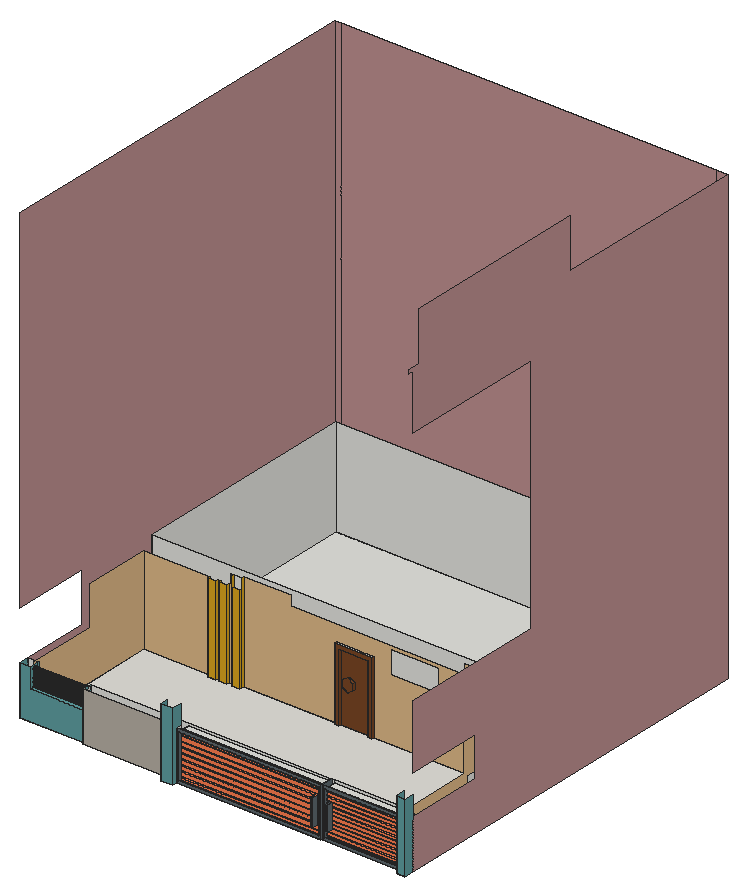
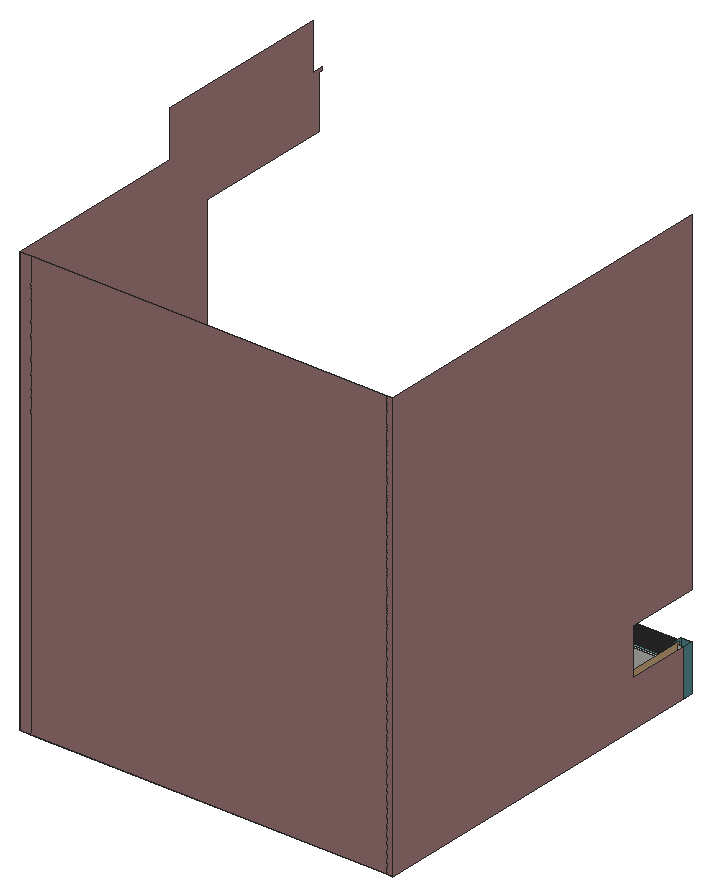
# SketchUp Ruby script. Lengths in inches.
U = 1.inch
M = Sketchup.active_model
def pt(a) = Geom::Point3d.new(a.map { |v| v * U })
def face(e, loops, mat)
  f = e.add_face(loops[0].map { |a| pt(a) })
  loops[1..].each { |l| e.add_face(l.map { |a| pt(a) }).erase! }
  f.material = f.back_material = mat if mat
  f
end
# faces: each face lists its corners as indices into pts; further lists are holes
def faces(e, pts, list, mat = nil) = list.each { |f| face(e, (f[0].is_a?(Array) ? f : [f]).map { |l| l.map { |i| pts[i] } }, mat) }
# xy, xz, yz: faces in a plane at the given z, y or x. An outline is a flat list of corners, or four numbers for a rectangle; further outlines are holes
def ring(l) = l.size == 4 ? [[l[0], l[1]], [l[2], l[1]], [l[2], l[3]], [l[0], l[3]]] : l.each_slice(2).to_a
def flat(e, list, mat, &to3) = list.each { |f| face(e, (f[0].is_a?(Array) ? f : [f]).map { |l| ring(l).map { |u, v| to3.(u, v) } }, mat) }
def xy(e, z, list, mat = nil) = flat(e, list, mat) { |x, y| [x, y, z] }
def xz(e, y, list, mat = nil) = flat(e, list, mat) { |x, z| [x, y, z] }
def yz(e, x, list, mat = nil) = flat(e, list, mat) { |y, z| [x, y, z] }
def lines(e, pts, list) = list.each { |a, b| e.add_line(pt(pts[a]), pt(pts[b])) }
# prism: a flat outline (further loops are holes) pulled along v
def prism(e, loops, v, mat = nil)
  f = face(e, loops, mat); d = Geom::Vector3d.new(v.map { |x| x * U })
  f.pushpull(f.normal.samedirection?(d) ? d.length : -d.length)
end
def box(e, o, s, mat = nil) = prism(e, [[o, [o[0] + s[0], o[1], o[2]], [o[0] + s[0], o[1] + s[1], o[2]], [o[0], o[1] + s[1], o[2]]]], [0, 0, s[2]], mat)
def at(x, y, z, deg = 0) = Geom::Transformation.translation(pt([x, y, z])) * Geom::Transformation.rotation(ORIGIN, Z_AXIS, deg.degrees)
def axes(o, x, y, z) = Geom::Transformation.new([*x, 0, *y, 0, *z, 0, *pt(o).to_a, 1])
def part(name) = M.definitions.add(name)
# library, detail: a bought-in or finely detailed component or shape, given as its bounding box
def library(name, o, s) = part(name).tap { |d| box(d.entities, o, s) }
def detail(e, o, s) = box(e.add_group.entities, o, s)
def put(e, d, t, mat = nil) = e.add_instance(d, t).tap { |i| i.material = mat if mat }
def group(e, t, mat = nil) = e.add_group.tap { |g| g.transformation = t; g.material = mat if mat }.entities
root = M.entities
M.materials.add("[0025_Coral]").color = [255, 127, 80]
M.materials.add("[0036_BurlyWood]").color = [222, 184, 135]
M.materials.add("[0045_Goldenrod]").color = [218, 165, 32]
M.materials.add("[0081_CadetBlue]").color = [95, 158, 160]
M.materials.add("[0119_RosyBrown]").color = [188, 143, 143]
M.materials.add("[Color M07]").color = [58, 58, 58]
M.materials.add("[Formica Speckled Grey]").color = [94, 105, 111]
M.materials.add("[Marble Carrara Gold Floor Tile]").color = [225, 223, 217]
M.materials.add("[Stone Masonry Multi]").color = [182, 175, 164]
M.materials.add("[Translucent Glass Blue]").color = [100, 149, 237]
M.materials["[Translucent Glass Blue]"].alpha = 0.5
M.materials.add("[Wood Floor Parquet]").color = [145, 89, 39]
M.materials.add("[Wood Veneer 01]").color = [120, 70, 37]
xy(root,0,[[181.875,0,195.69,12],[469.21,0,471,12],[471,0,480,12],[373.99,6,374.05,12],[79.49,9,181.875,11.375],
  [79.49,11.375,181.875,12],[0,12,79.49,24.5],[372.4375,12,373.99,21],[373.99,12,376.99,21],[466.21,12,466.21,21,471,21,471,18.5625,469.21,18.5625,469.21,12],
  [469.21,12,471,18.5625],[471,12,480,18.5625],[471,18.5625,480,106.65],[0,24.5,9,106.65],[0,106.65,7.75,492],
  [7.75,106.65,7.75,492,466.21,492,466.21,483,9,483,9,201.23,466.21,201.23,466.21,192.3,129,192.3,129,189.3,113.21,189.3,113.21,186.3,103.48,186.3,103.48,189.3,99.83,189.3,99.83,186.3,90.1,186.3,90.1,189.3,9,189.3,9,106.65],[466.21,106.65,471,192.3],[471,106.65,471,483,466.21,483,466.21,492,480,492,480,106.65],[118.73,186.3,128.46,189.3],[242.24,189.3,246.91,192.3],
  [282.91,189.3,287.58,192.3],[466.21,192.3,471,201.23],[9,201.23,466.21,483],[466.21,201.23,471,203.34],[466.21,203.34,471,483]])
xy(root,0,[[195.69,6,372.4375,12],[374.05,6,469.21,12],[79.49,12,372.4375,21],[376.99,12,466.21,21]],"[Formica Speckled Grey]")
xy(root,0,[[79.49,21,466.21,21,466.21,192.3,287.58,192.3,287.58,189.3,282.91,189.3,282.91,192.3,246.91,192.3,246.91,189.3,242.24,189.3,242.24,192.3,129,192.3,129,189.3,128.46,189.3,128.46,186.3,118.73,186.3,118.73,189.3,113.21,189.3,113.21,186.3,103.48,186.3,103.48,189.3,99.83,189.3,99.83,186.3,90.1,186.3,90.1,189.3,9,189.3,9,24.5,79.49,24.5]],"[Marble Carrara Gold Floor Tile]")
xy(root,3,[[198.69,9,369.4375,12],[376.99,9,466.21,12],[198.69,12,369.4375,21],[376.99,12,466.21,21],[466.21,12,466.21,21,471,21,471,18.5625,469.21,18.5625,469.21,12],
  [469.21,12,469.21,18.5625,471,18.5625,471,21,473.21,21,473.21,12],[466.21,21,471,203.34]])
xy(root,3,[[198.69,6,369.4375,9],[376.99,6,466.21,9]],"[Formica Speckled Grey]")
xy(root,3.875,[[376.99,9,466.21,12]],"[0025_Coral]")
xy(root,5.28,[[376.99,9,466.21,12]])
xy(root,5.5,[[198.69,9,369.4375,12]],"[0025_Coral]")
xy(root,7.31,[[198.69,9,369.4375,12]],"[0025_Coral]")
xy(root,8.6875,[[376.99,9,466.21,12]],"[0025_Coral]")
xy(root,10.09,[[376.99,9,466.21,12]],"[0025_Coral]")
xy(root,11.62,[[362.15,3,364.83,9]],"[Formica Speckled Grey]")
xy(root,11.9375,[[198.69,9,369.4375,12]],"[0025_Coral]")
xy(root,13.5,[[376.99,9,466.21,12]],"[0025_Coral]")
xy(root,13.53,[[381.11,3,383.59,9]],"[Formica Speckled Grey]")
xy(root,13.75,[[198.69,9,369.4375,12]],"[0025_Coral]")
xy(root,14.9,[[376.99,9,466.21,12]],"[0025_Coral]")
xy(root,18.3125,[[376.99,9,466.21,12]],"[0025_Coral]")
xy(root,18.375,[[198.69,9,369.4375,12]],"[0025_Coral]")
xy(root,19.71,[[376.99,9,466.21,12]],"[0025_Coral]")
xy(root,20.18,[[198.69,9,369.4375,12]],"[0025_Coral]")
xy(root,23.125,[[376.99,9,466.21,12]],"[0025_Coral]")
xy(root,24.53,[[376.99,9,466.21,12]],"[0025_Coral]")
xy(root,24.8125,[[198.69,9,369.4375,12]],"[0025_Coral]")
xy(root,26.62,[[198.69,9,369.4375,12]],"[0025_Coral]")
xy(root,27.9375,[[376.99,9,466.21,12]],"[0025_Coral]")
xy(root,29.34,[[376.99,9,466.21,12]],"[0025_Coral]")
xy(root,31.25,[[198.69,9,369.4375,12]],"[0025_Coral]")
xy(root,32.75,[[376.99,9,466.21,12]],"[0025_Coral]")
xy(root,33.06,[[198.69,9,369.4375,12]],"[0025_Coral]")
xy(root,34.15,[[376.99,9,466.21,12]],"[0025_Coral]")
xy(root,35.625,[[12.93,21,79.49,24.5]])
xy(root,35.625,[[12.93,12,79.49,21]],"[0081_CadetBlue]")
xy(root,37.5625,[[376.99,9,466.21,12]],"[0025_Coral]")
xy(root,37.6875,[[198.69,9,369.4375,12]],"[0025_Coral]")
xy(root,38.96,[[376.99,9,466.21,12]],"[0025_Coral]")
xy(root,39.5,[[198.69,9,369.4375,12]],"[0025_Coral]")
xy(root,42.375,[[381.11,3,383.59,3,383.59,9,466.21,9,466.21,12,376.99,12,376.99,9,381.11,9]],"[0025_Coral]")
xy(root,43.78,[[376.99,9,466.21,12]],"[0025_Coral]")
xy(root,44.125,[[362.15,3,364.83,3,364.83,9,369.4375,9,369.4375,12,198.69,12,198.69,9,362.15,9]],"[0025_Coral]")
xy(root,44.1875,[[410.91,189.3,442.47,192.3]],"[Wood Floor Parquet]")
xy(root,45.93,[[198.69,9,369.4375,12]],"[0025_Coral]")
xy(root,47.1875,[[376.99,9,466.21,12]],"[0025_Coral]")
xy(root,47.1875,[[413.91,189.3,439.47,192.3]],"[Wood Floor Parquet]")
xy(root,48.59,[[376.99,9,466.21,12]],"[0025_Coral]")
xy(root,50.5625,[[198.69,9,369.4375,12]],"[0025_Coral]")
xy(root,52,[[376.99,9,466.21,12]],"[0025_Coral]")
xy(root,52.37,[[198.69,9,369.4375,12]],"[0025_Coral]")
xy(root,53.59,[[376.99,9,466.21,12]],"[0025_Coral]")
xy(root,57,[[198.69,9,369.4375,12],[376.99,9,466.21,12],[198.69,12,369.4375,21],[376.99,12,466.21,21],[466.21,12,473.21,21]])
xy(root,57,[[198.69,6,369.4375,9],[376.99,6,466.21,9]],"[Formica Speckled Grey]")
xz(root,0,[[181.875,0,195.69,84],[469.21,0,480,84]],"[0081_CadetBlue]")
xz(root,3,[[362.15,11.62,364.83,44.125],[381.11,13.53,383.59,42.375]],"[Formica Speckled Grey]")
xz(root,6,[[373.99,0,374.05,60]])
xz(root,6,[[[195.69,0,372.4375,60],[198.69,3,369.4375,57]],[[374.05,0,469.21,60],[376.99,3,466.21,57]]],"[Formica Speckled Grey]")
xz(root,9,[[362.15,11.62,364.83,11.9375],[362.15,11.9375,364.83,13.75],[381.11,13.5,383.59,13.53],[381.11,13.53,383.59,14.9],[362.15,13.75,364.83,18.375],
  [381.11,14.9,383.59,18.3125],[381.11,18.3125,383.59,19.71],[362.15,18.375,364.83,20.18],[381.11,19.71,383.59,23.125],[362.15,20.18,364.83,24.8125],
  [381.11,23.125,383.59,24.53],[381.11,24.53,383.59,27.9375],[362.15,24.8125,364.83,26.62],[362.15,26.62,364.83,31.25],[381.11,27.9375,383.59,29.34],
  [381.11,29.34,383.59,32.75],[362.15,31.25,364.83,33.06],[381.11,32.75,383.59,34.15],[362.15,33.06,364.83,37.6875],[381.11,34.15,383.59,37.5625],
  [381.11,37.5625,383.59,38.96],[362.15,37.6875,364.83,39.5]])
xz(root,9,[[198.69,3,369.4375,5.5],[376.99,3,466.21,3.875],[376.99,5.28,466.21,8.6875],[198.69,7.31,369.4375,7.31,369.4375,11.9375,364.83,11.9375,364.83,11.62,362.15,11.62,362.15,11.9375,198.69,11.9375],[376.99,10.09,466.21,13.5],
  [198.69,13.75,362.15,18.375],[364.83,13.75,369.4375,18.375],[376.99,14.9,381.11,18.3125],[383.59,14.9,466.21,18.3125],[376.99,19.71,381.11,23.125],
  [383.59,19.71,466.21,23.125],[198.69,20.18,362.15,24.8125],[364.83,20.18,369.4375,24.8125],[376.99,24.53,381.11,27.9375],[383.59,24.53,466.21,27.9375],
  [198.69,26.62,362.15,31.25],[364.83,26.62,369.4375,31.25],[376.99,29.34,381.11,32.75],[383.59,29.34,466.21,32.75],[198.69,33.06,362.15,37.6875],
  [364.83,33.06,369.4375,37.6875],[376.99,34.15,381.11,37.5625],[383.59,34.15,466.21,37.5625],[376.99,38.96,381.11,42.375],[383.59,38.96,466.21,42.375],
  [198.69,39.5,362.15,44.125],[364.83,39.5,369.4375,44.125],[376.99,43.78,466.21,47.1875],[198.69,45.93,369.4375,50.5625],[376.99,48.59,466.21,52],
  [198.69,52.37,369.4375,57],[376.99,53.59,466.21,57]],"[0025_Coral]")
xz(root,9,[[79.49,0,181.875,60]],"[Stone Masonry Multi]")
xz(root,12,[[181.875,0,195.69,60],[376.99,0,466.21,0.46],[466.21,0,469.21,3],[469.21,0,480,0,480,60,469.21,60,469.21,57,473.21,57,473.21,3,469.21,3],[376.99,0.46,466.21,3],
  [198.69,0.87,369.4375,3],[198.69,3,369.4375,5.5],[376.99,3,466.21,3.875],[466.21,3,469.21,3.875],[469.21,3,473.21,3.875],
  [466.21,3.875,469.21,5.28],[469.21,3.875,473.21,5.28],[376.99,5.28,466.21,8.6875],[466.21,5.28,469.21,8.6875],[469.21,5.28,473.21,8.6875],
  [198.69,7.31,369.4375,11.9375],[466.21,8.6875,469.21,10.09],[469.21,8.6875,473.21,10.09],[376.99,10.09,466.21,13.5],[466.21,10.09,469.21,13.5],
  [469.21,10.09,473.21,13.5],[466.21,13.5,469.21,14.9],[469.21,13.5,473.21,14.9],[198.69,13.75,369.4375,18.375],[376.99,14.9,466.21,18.3125],
  [466.21,14.9,469.21,18.3125],[469.21,14.9,473.21,18.3125],[466.21,18.3125,469.21,19.71],[469.21,18.3125,473.21,19.71],[376.99,19.71,466.21,23.125],
  [466.21,19.71,469.21,23.125],[469.21,19.71,473.21,23.125],[198.69,20.18,369.4375,24.8125],[466.21,23.125,469.21,24.53],[469.21,23.125,473.21,24.53],
  [376.99,24.53,466.21,27.9375],[466.21,24.53,469.21,27.9375],[469.21,24.53,473.21,27.9375],[198.69,26.62,369.4375,31.25],[466.21,27.9375,469.21,29.34],
  [469.21,27.9375,473.21,29.34],[376.99,29.34,466.21,32.75],[466.21,29.34,469.21,32.75],[469.21,29.34,473.21,32.75],[466.21,32.75,469.21,34.15],
  [469.21,32.75,473.21,34.15],[198.69,33.06,369.4375,37.6875],[376.99,34.15,466.21,37.5625],[466.21,34.15,469.21,37.5625],[469.21,34.15,473.21,37.5625],
  [466.21,37.5625,469.21,38.96],[469.21,37.5625,473.21,38.96],[376.99,38.96,466.21,42.375],[466.21,38.96,469.21,42.375],[469.21,38.96,473.21,42.375],
  [198.69,39.5,369.4375,44.125],[466.21,42.375,469.21,43.78],[469.21,42.375,473.21,43.78],[376.99,43.78,466.21,47.1875],[466.21,43.78,469.21,47.1875],
  [469.21,43.78,473.21,47.1875],[198.69,45.93,369.4375,50.5625],[466.21,47.1875,469.21,48.59],[469.21,47.1875,473.21,48.59],[376.99,48.59,466.21,52],
  [466.21,48.59,469.21,52],[469.21,48.59,473.21,52],[466.21,52,469.21,53.59],[469.21,52,473.21,53.59],[198.69,52.37,369.4375,57],
  [376.99,53.59,466.21,57],[466.21,53.59,469.21,57],[469.21,53.59,473.21,57],[466.21,57,469.21,60]])
xz(root,12,[[0,0,79.49,0,79.49,35.625,12.93,35.625,12.93,60,0,60]],"[0081_CadetBlue]")
xz(root,18.5625,[[469.21,0,471,3]])
xz(root,21,[[[79.49,0,372.4375,60],[198.69,3,369.4375,57]],[373.99,0,376.99,60],[376.99,0,466.21,3],[466.21,0,471,3],[471,3,473.21,57],
  [376.99,57,466.21,60]])
xz(root,24.5,[[0,0,0,60,12.93,60,12.93,35.625,79.49,35.625,79.49,0]])
xz(root,186.3,[[90.1,0,99.83,108],[103.48,0,113.21,108],[118.73,0,128.46,108]],"[0045_Goldenrod]")
xz(root,189.3,[[118.73,0,128.46,120]])
xz(root,189.3,[[9,0,90.1,108],[99.83,0,103.48,108],[113.21,0,118.73,0,118.73,120,115.97,120,115.97,108,113.21,108]],"[0036_BurlyWood]")
xz(root,189.3,[[128.46,0,129,108]],"[0045_Goldenrod]")
xz(root,189.3,[[[410.91,44.1875,442.47,44.1875,442.47,108,418.65,108,418.65,108.6875,416.3125,108.6875,416.3125,108,410.91,108],[413.91,47.1875,439.47,105.6875]]],"[Wood Floor Parquet]")
xz(root,189.3,[[242.24,0,246.91,0,246.91,84,282.91,84,282.91,0,287.58,0,287.58,88.67,242.24,88.67],[258.125,39.92,264.94,43.86,264.94,51.73,258.125,55.67,251.3,51.73,251.3,43.86]],"[Wood Veneer 01]")
xz(root,192.3,[[242.24,0,242.24,88.67,287.58,88.67,287.58,0,282.91,0,282.91,84,246.91,84,246.91,0]])
xz(root,192.3,[[[129,0,242.24,0,242.24,88.67,287.58,88.67,287.58,0,466.21,0,466.21,108,458.79,108,458.79,120,398.79,120,398.79,108,186.5,108,186.5,120,129,120],[410.91,44.1875,442.47,108.6875],[308.99,75.62,366.74,104.31]]],"[0036_BurlyWood]")
xz(root,192.3,[[413.91,47.1875,439.47,105.6875]],"[Translucent Glass Blue]")
xz(root,192.3,[[[246.91,0,282.91,84],[258.125,39.92,251.3,43.86,251.3,51.73,258.125,55.67,264.94,51.73,264.94,43.86]]],"[Wood Veneer 01]")
xz(root,201.23,[[9,0,471,120]])
xz(root,203.34,[[466.21,0,471,3]])
xz(root,483,[[9,0,471,120]])
xz(root,492,[[0,0,7.75,552],[7.75,0,466.21,552],[466.21,0,480,552]],"[0119_RosyBrown]")
yz(root,0,[[12,0,24.5,60]],"[0081_CadetBlue]")
yz(root,0,[[24.5,0,24.5,60,106.65,60,106.65,120,12,120,12,552,492,552,492,0]],"[0119_RosyBrown]")
yz(root,9,[[201.23,0,483,120]])
yz(root,9,[[21,0,189.3,0,189.3,108,106.65,108,106.65,60,21,60]],"[0036_BurlyWood]")
yz(root,12.93,[[16.84,31.14,17.32,31.2,17.77,31.39,18.16,31.6875,18.46,32.07,18.65,32.53,18.71,33.01,18.65,33.5,18.46,33.95,18.16,34.34,17.77,34.64,17.32,34.82,16.84,34.89,16.35,34.82,15.9,34.64,15.51,34.34,15.21,33.95,15.03,33.5,14.96,33.01,15.03,32.53,15.21,32.07,15.51,31.6875,15.9,31.39,16.35,31.2]])
yz(root,12.93,[[[12,35.625,21,60],[16.84,50.39,16.35,50.45,15.9,50.64,15.51,50.9375,15.21,51.32,15.03,51.78,14.96,52.26,15.03,52.75,15.21,53.2,15.51,53.59,15.9,53.89,16.35,54.07,16.84,54.14,17.32,54.07,17.77,53.89,18.16,53.59,18.46,53.2,18.65,52.75,18.71,52.26,18.65,51.78,18.46,51.32,18.16,50.9375,17.77,50.64,17.32,50.45],[16.84,45.57,16.35,45.64,15.9,45.83,15.51,46.125,15.21,46.51,15.03,46.96,14.96,47.45,15.03,47.94,15.21,48.39,15.51,48.78,15.9,49.07,16.35,49.26,16.84,49.32,17.32,49.26,17.77,49.07,18.16,48.78,18.46,48.39,18.65,47.94,18.71,47.45,18.65,46.96,18.46,46.51,18.16,46.125,17.77,45.83,17.32,45.64],[16.84,40.76,16.35,40.83,15.9,41.01,15.51,41.3125,15.21,41.7,15.03,42.15,14.96,42.64,15.03,43.12,15.21,43.57,15.51,43.96,15.9,44.26,16.35,44.45,16.84,44.51,17.32,44.45,17.77,44.26,18.16,43.96,18.46,43.57,18.65,43.12,18.71,42.64,18.65,42.15,18.46,41.7,18.16,41.3125,17.77,41.01,17.32,40.83],[16.84,35.95,16.35,36.01,15.9,36.2,15.51,36.5,15.21,36.89,15.03,37.34,14.96,37.82,15.03,38.31,15.21,38.76,15.51,39.15,15.9,39.45,16.35,39.64,16.84,39.7,17.32,39.64,17.77,39.45,18.16,39.15,18.46,38.76,18.65,38.31,18.71,37.82,18.65,37.34,18.46,36.89,18.16,36.5,17.77,36.2,17.32,36.01],[16.84,55.2,16.35,55.26,15.9,55.45,15.51,55.75,15.21,56.14,15.03,56.59,14.96,57.07,15.03,57.56,15.21,58.01,15.51,58.4,15.9,58.7,16.35,58.89,16.84,58.95,17.32,58.89,17.77,58.7,18.16,58.4,18.46,58.01,18.65,57.56,18.71,57.07,18.65,56.59,18.46,56.14,18.16,55.75,17.77,55.45,17.32,55.26]],[21,35.625,24.5,60]],"[0081_CadetBlue]")
yz(root,79.43,[[16.84,45.57,17.32,45.64,17.77,45.83,18.16,46.125,18.46,46.51,18.65,46.96,18.71,47.45,18.65,47.94,18.46,48.39,18.16,48.78,17.77,49.07,17.32,49.26,16.84,49.32,16.35,49.26,15.9,49.07,15.51,48.78,15.21,48.39,15.03,47.94,14.96,47.45,15.03,46.96,15.21,46.51,15.51,46.125,15.9,45.83,16.35,45.64]])
yz(root,79.49,[[12,0,21,35.625],[21,0,24.5,35.625]])
yz(root,79.49,[[12,35.625,21,60]],"[0081_CadetBlue]")
yz(root,79.49,[[9,0,12,60]],"[Stone Masonry Multi]")
yz(root,79.55,[[16.84,40.76,17.32,40.83,17.77,41.01,18.16,41.3125,18.46,41.7,18.65,42.15,18.71,42.64,18.65,43.12,18.46,43.57,18.16,43.96,17.77,44.26,17.32,44.45,16.84,44.51,16.35,44.45,15.9,44.26,15.51,43.96,15.21,43.57,15.03,43.12,14.96,42.64,15.03,42.15,15.21,41.7,15.51,41.3125,15.9,41.01,16.35,40.83]])
yz(root,79.68,[[16.84,55.2,17.32,55.26,17.77,55.45,18.16,55.75,18.46,56.14,18.65,56.59,18.71,57.07,18.65,57.56,18.46,58.01,18.16,58.4,17.77,58.7,17.32,58.89,16.84,58.95,16.35,58.89,15.9,58.7,15.51,58.4,15.21,58.01,15.03,57.56,14.96,57.07,15.03,56.59,15.21,56.14,15.51,55.75,15.9,55.45,16.35,55.26]])
yz(root,80.62,[[16.84,35.95,17.32,36.01,17.77,36.2,18.16,36.5,18.46,36.89,18.65,37.34,18.71,37.82,18.65,38.31,18.46,38.76,18.16,39.15,17.77,39.45,17.32,39.64,16.84,39.7,16.35,39.64,15.9,39.45,15.51,39.15,15.21,38.76,15.03,38.31,14.96,37.82,15.03,37.34,15.21,36.89,15.51,36.5,15.9,36.2,16.35,36.01]])
yz(root,90.1,[[186.3,0,189.3,108]],"[0045_Goldenrod]")
yz(root,99.83,[[186.3,0,189.3,108]],"[0045_Goldenrod]")
yz(root,103.48,[[186.3,0,189.3,108]],"[0045_Goldenrod]")
yz(root,113.21,[[186.3,0,189.3,108]],"[0045_Goldenrod]")
yz(root,118.73,[[186.3,0,189.3,120]],"[0045_Goldenrod]")
yz(root,128.46,[[186.3,0,189.3,108]],"[0045_Goldenrod]")
yz(root,129,[[189.3,0,192.3,120]],"[0045_Goldenrod]")
yz(root,181.875,[[9,0,11.375,60],[11.375,0,12,60]])
yz(root,181.875,[[0,0,9,84]],"[0081_CadetBlue]")
yz(root,195.69,[[6,0,12,60]])
yz(root,195.69,[[0,0,6,0,6,60,12,60,12,84,0,84]],"[0081_CadetBlue]")
yz(root,198.69,[[9,3,12,5.5],[12,3,21,57],[9,7.31,12,11.9375],[9,13.75,12,18.375],[9,20.18,12,24.8125],
  [9,26.62,12,31.25],[9,33.06,12,37.6875],[9,39.5,12,44.125],[9,45.93,12,50.5625],[9,52.37,12,57]])
yz(root,198.69,[[6,3,9,3,9,5.5,12,5.5,12,7.31,9,7.31,9,11.9375,12,11.9375,12,13.75,9,13.75,9,18.375,12,18.375,12,20.18,9,20.18,9,24.8125,12,24.8125,12,26.62,9,26.62,9,31.25,12,31.25,12,33.06,9,33.06,9,37.6875,12,37.6875,12,39.5,9,39.5,9,44.125,12,44.125,12,45.93,9,45.93,9,50.5625,12,50.5625,12,52.37,9,52.37,9,57,6,57]],"[Formica Speckled Grey]")
yz(root,242.24,[[189.3,0,192.3,88.67]],"[Wood Veneer 01]")
yz(root,246.91,[[189.3,0,192.3,84]],"[Wood Veneer 01]")
yz(root,251.3,[[189.3,43.86,192.3,51.73]],"[Wood Veneer 01]")
yz(root,264.94,[[189.3,43.86,192.3,51.73]],"[Wood Veneer 01]")
yz(root,282.91,[[189.3,0,192.3,84]],"[Wood Veneer 01]")
yz(root,287.58,[[189.3,0,192.3,88.67]],"[Wood Veneer 01]")
yz(root,362.15,[[3,11.62,9,44.125]],"[Formica Speckled Grey]")
yz(root,364.83,[[3,11.62,9,44.125]],"[Formica Speckled Grey]")
yz(root,369.4375,[[9,3,12,5.5],[12,3,21,57],[9,7.31,12,11.9375],[9,13.75,12,18.375],[9,20.18,12,24.8125],
  [9,26.62,12,31.25],[9,33.06,12,37.6875],[9,39.5,12,44.125],[9,45.93,12,50.5625],[9,52.37,12,57]])
yz(root,369.4375,[[6,3,6,57,9,57,9,52.37,12,52.37,12,50.5625,9,50.5625,9,45.93,12,45.93,12,44.125,9,44.125,9,39.5,12,39.5,12,37.6875,9,37.6875,9,33.06,12,33.06,12,31.25,9,31.25,9,26.62,12,26.62,12,24.8125,9,24.8125,9,20.18,12,20.18,12,18.375,9,18.375,9,13.75,12,13.75,12,11.9375,9,11.9375,9,7.31,12,7.31,12,5.5,9,5.5,9,3]],"[Formica Speckled Grey]")
yz(root,372.4375,[[6,0,21,60]],"[Formica Speckled Grey]")
yz(root,373.99,[[6,0,21,60]],"[Formica Speckled Grey]")
yz(root,376.99,[[12,0,21,3],[9,3,12,3.875],[12,3,21,57],[9,5.28,12,8.6875],[9,10.09,12,13.5],
  [9,14.9,12,18.3125],[9,19.71,12,23.125],[9,24.53,12,27.9375],[9,29.34,12,32.75],[9,34.15,12,37.5625],
  [9,38.96,12,42.375],[9,43.78,12,47.1875],[9,48.59,12,52],[9,53.59,12,57]])
yz(root,376.99,[[6,3,9,3,9,3.875,12,3.875,12,5.28,9,5.28,9,8.6875,12,8.6875,12,10.09,9,10.09,9,13.5,12,13.5,12,14.9,9,14.9,9,18.3125,12,18.3125,12,19.71,9,19.71,9,23.125,12,23.125,12,24.53,9,24.53,9,27.9375,12,27.9375,12,29.34,9,29.34,9,32.75,12,32.75,12,34.15,9,34.15,9,37.5625,12,37.5625,12,38.96,9,38.96,9,42.375,12,42.375,12,43.78,9,43.78,9,47.1875,12,47.1875,12,48.59,9,48.59,9,52,12,52,12,53.59,9,53.59,9,57,6,57]],"[Formica Speckled Grey]")
yz(root,381.11,[[3,13.53,9,42.375]],"[Formica Speckled Grey]")
yz(root,383.59,[[3,13.53,9,42.375]],"[Formica Speckled Grey]")
yz(root,410.91,[[189.3,44.1875,192.3,108.6875]],"[Wood Floor Parquet]")
yz(root,413.91,[[189.3,47.1875,192.3,105.6875]],"[Wood Floor Parquet]")
yz(root,439.47,[[189.3,47.1875,192.3,105.6875]],"[Wood Floor Parquet]")
yz(root,442.47,[[189.3,44.1875,192.3,108.6875]],"[Wood Floor Parquet]")
yz(root,466.21,[[12,0,21,3],[21,0,106.65,3],[106.65,0,192.3,3],[192.3,0,203.34,3],[9,3,12,3.875],
  [9,5.28,12,8.6875],[9,10.09,12,13.5],[9,14.9,12,18.3125],[9,19.71,12,23.125],[9,24.53,12,27.9375],
  [9,29.34,12,32.75],[9,34.15,12,37.5625],[9,38.96,12,42.375],[9,43.78,12,47.1875],[9,48.59,12,52],
  [9,53.59,12,57]])
yz(root,466.21,[[12,3,12,57,21,57,21,60,106.65,60,106.65,108,192.3,108,192.3,3]],"[0036_BurlyWood]")
yz(root,466.21,[[6,3,6,57,9,57,9,53.59,12,53.59,12,52,9,52,9,48.59,12,48.59,12,47.1875,9,47.1875,9,43.78,12,43.78,12,42.375,9,42.375,9,38.96,12,38.96,12,37.5625,9,37.5625,9,34.15,12,34.15,12,32.75,9,32.75,9,29.34,12,29.34,12,27.9375,9,27.9375,9,24.53,12,24.53,12,23.125,9,23.125,9,19.71,12,19.71,12,18.3125,9,18.3125,9,14.9,12,14.9,12,13.5,9,13.5,9,10.09,12,10.09,12,8.6875,9,8.6875,9,5.28,12,5.28,12,3.875,9,3.875,9,3]],"[Formica Speckled Grey]")
yz(root,469.21,[[6,0,12,60],[12,0,18.5625,3]])
yz(root,469.21,[[0,0,0,84,12,84,12,60,6,60,6,0]],"[0081_CadetBlue]")
yz(root,471,[[18.5625,0,21,3],[21,0,106.65,3],[106.65,0,192.3,3],[192.3,0,201.23,3],[201.23,0,203.34,3],
  [203.34,0,203.34,3,201.23,3,201.23,120,483,120,483,0],[106.65,3,192.3,60]])
yz(root,473.21,[[12,3,21,57]])
yz(root,480,[[0,0,12,84]],"[0081_CadetBlue]")
yz(root,480,[[12,0,492,0,492,552,251.9375,552,251.9375,612,21,612,21,552,5.9375,552,5.9375,547.59,12,547.59,12,480,192.3,480,192.3,186.25,12,186.25,12,108,106.65,108,106.65,60,12,60]],"[0119_RosyBrown]")
p = [[12.93,16.35,36.01],[12.93,16.84,35.95],[80.62,16.84,35.95],[80.62,16.35,36.01],[12.93,17.32,36.01],[80.62,17.32,36.01],
  [12.93,15.9,36.2],[80.62,15.9,36.2],[12.93,17.77,36.2],[80.62,17.77,36.2],[12.93,15.51,36.5],[80.62,15.51,36.5],
  [12.93,18.16,36.5],[80.62,18.16,36.5],[12.93,15.21,36.89],[80.62,15.21,36.89],[12.93,18.46,36.89],[80.62,18.46,36.89],
  [12.93,15.03,37.34],[80.62,15.03,37.34],[12.93,18.65,37.34],[80.62,18.65,37.34],[12.93,14.96,37.82],[80.62,14.96,37.82],
  [12.93,18.71,37.82],[80.62,18.71,37.82],[12.93,15.03,38.31],[80.62,15.03,38.31],[12.93,18.65,38.31],[80.62,18.65,38.31],
  [12.93,15.21,38.76],[80.62,15.21,38.76],[12.93,18.46,38.76],[80.62,18.46,38.76],[12.93,15.51,39.15],[80.62,15.51,39.15],
  [12.93,18.16,39.15],[80.62,18.16,39.15],[12.93,15.9,39.45],[80.62,15.9,39.45],[12.93,17.77,39.45],[80.62,17.77,39.45],
  [12.93,16.35,39.64],[80.62,16.35,39.64],[12.93,17.32,39.64],[80.62,17.32,39.64],[12.93,16.84,39.7],[80.62,16.84,39.7],
  [251.3,192.3,43.86],[258.125,192.3,39.92],[258.125,189.3,39.92],[251.3,189.3,43.86],[264.94,192.3,43.86],[264.94,189.3,43.86],
  [12.93,15.9,41.01],[12.93,16.35,40.83],[79.55,16.35,40.83],[79.55,15.9,41.01],[12.93,16.84,40.76],[79.55,16.84,40.76],
  [12.93,17.32,40.83],[79.55,17.32,40.83],[12.93,17.77,41.01],[79.55,17.77,41.01],[12.93,15.51,41.3125],[79.55,15.51,41.3125],
  [12.93,18.16,41.3125],[79.55,18.16,41.3125],[12.93,15.21,41.7],[79.55,15.21,41.7],[12.93,18.46,41.7],[79.55,18.46,41.7],
  [12.93,15.03,42.15],[79.55,15.03,42.15],[12.93,18.65,42.15],[79.55,18.65,42.15],[12.93,14.96,42.64],[79.55,14.96,42.64],
  [12.93,18.71,42.64],[79.55,18.71,42.64],[12.93,15.03,43.12],[79.55,15.03,43.12],[12.93,18.65,43.12],[79.55,18.65,43.12],
  [12.93,15.21,43.57],[79.55,15.21,43.57],[12.93,18.46,43.57],[79.55,18.46,43.57],[12.93,15.51,43.96],[79.55,15.51,43.96],
  [12.93,18.16,43.96],[79.55,18.16,43.96],[12.93,15.9,44.26],[79.55,15.9,44.26],[12.93,17.77,44.26],[79.55,17.77,44.26],
  [12.93,16.35,44.45],[79.55,16.35,44.45],[12.93,17.32,44.45],[79.55,17.32,44.45],[12.93,16.84,44.51],[79.55,16.84,44.51],
  [12.93,15.9,45.83],[12.93,16.35,45.64],[79.43,16.35,45.64],[79.43,15.9,45.83],[12.93,16.84,45.57],[79.43,16.84,45.57],
  [12.93,17.32,45.64],[79.43,17.32,45.64],[12.93,17.77,45.83],[79.43,17.77,45.83],[12.93,15.51,46.125],[79.43,15.51,46.125],
  [12.93,18.16,46.125],[79.43,18.16,46.125],[12.93,15.21,46.51],[79.43,15.21,46.51],[12.93,18.46,46.51],[79.43,18.46,46.51],
  [12.93,15.03,46.96],[79.43,15.03,46.96],[12.93,18.65,46.96],[79.43,18.65,46.96],[12.93,14.96,47.45],[79.43,14.96,47.45],
  [12.93,18.71,47.45],[79.43,18.71,47.45],[12.93,15.03,47.94],[79.43,15.03,47.94],[12.93,18.65,47.94],[79.43,18.65,47.94],
  [12.93,15.21,48.39],[79.43,15.21,48.39],[12.93,18.46,48.39],[79.43,18.46,48.39],[12.93,15.51,48.78],[79.43,15.51,48.78],
  [12.93,18.16,48.78],[79.43,18.16,48.78],[12.93,15.9,49.07],[79.43,15.9,49.07],[12.93,17.77,49.07],[79.43,17.77,49.07],
  [12.93,16.35,49.26],[79.43,16.35,49.26],[12.93,17.32,49.26],[79.43,17.32,49.26],[12.93,16.84,49.32],[79.43,16.84,49.32],
  [12.93,16.35,50.45],[12.93,16.84,50.39],[79.49,16.84,50.39],[79.49,16.35,50.45],[12.93,17.32,50.45],[79.49,17.32,50.45],
  [12.93,15.9,50.64],[79.49,15.9,50.64],[12.93,17.77,50.64],[79.49,17.77,50.64],[12.93,15.51,50.9375],[79.49,15.51,50.9375],
  [12.93,18.16,50.9375],[79.49,18.16,50.9375],[12.93,15.21,51.32],[79.49,15.21,51.32],[12.93,18.46,51.32],[79.49,18.46,51.32],
  [12.93,15.03,51.78],[79.49,15.03,51.78],[12.93,18.65,51.78],[79.49,18.65,51.78],[258.125,192.3,55.67],[251.3,192.3,51.73],
  [251.3,189.3,51.73],[258.125,189.3,55.67],[264.94,192.3,51.73],[264.94,189.3,51.73],[12.93,14.96,52.26],[79.49,14.96,52.26],
  [12.93,18.71,52.26],[79.49,18.71,52.26],[12.93,15.03,52.75],[79.49,15.03,52.75],[12.93,18.65,52.75],[79.49,18.65,52.75],
  [12.93,15.21,53.2],[79.49,15.21,53.2],[12.93,18.46,53.2],[79.49,18.46,53.2],[12.93,15.51,53.59],[79.49,15.51,53.59],
  [12.93,18.16,53.59],[79.49,18.16,53.59],[12.93,15.9,53.89],[79.49,15.9,53.89],[12.93,17.77,53.89],[79.49,17.77,53.89],
  [12.93,16.35,54.07],[79.49,16.35,54.07],[12.93,17.32,54.07],[79.49,17.32,54.07],[12.93,16.84,54.14],[79.49,16.84,54.14],
  [12.93,16.35,55.26],[12.93,16.84,55.2],[79.68,16.84,55.2],[79.68,16.35,55.26],[12.93,17.32,55.26],[79.68,17.32,55.26],
  [12.93,15.9,55.45],[79.68,15.9,55.45],[12.93,17.77,55.45],[79.68,17.77,55.45],[12.93,15.51,55.75],[79.68,15.51,55.75],
  [12.93,18.16,55.75],[79.68,18.16,55.75],[12.93,15.21,56.14],[79.68,15.21,56.14],[12.93,18.46,56.14],[79.68,18.46,56.14],
  [12.93,15.03,56.59],[79.68,15.03,56.59],[12.93,18.65,56.59],[79.68,18.65,56.59],[12.93,14.96,57.07],[79.68,14.96,57.07],
  [12.93,18.71,57.07],[79.68,18.71,57.07],[12.93,15.03,57.56],[79.68,15.03,57.56],[12.93,18.65,57.56],[79.68,18.65,57.56],
  [12.93,15.21,58.01],[79.68,15.21,58.01],[12.93,18.46,58.01],[79.68,18.46,58.01],[12.93,15.51,58.4],[79.68,15.51,58.4],
  [12.93,18.16,58.4],[79.68,18.16,58.4],[12.93,15.9,58.7],[79.68,15.9,58.7],[12.93,17.77,58.7],[79.68,17.77,58.7],
  [12.93,16.35,58.89],[79.68,16.35,58.89],[12.93,17.32,58.89],[79.68,17.32,58.89],[12.93,16.84,58.95],[79.68,16.84,58.95],
  [282.91,196.8,0],[282.91,196.8,84],[246.91,196.8,84],[246.91,196.8,0],[7.75,106.65,0],[7.75,106.65,60],
  [376.99,12,60],[376.99,12,57],[469.21,18.5625,60],[469.21,18.5625,3],[471,21,60],[471,21,57]]
faces(root,p,[[0,1,2,3],[1,4,5,2],[6,0,3,7],[4,8,9,5],[10,6,7,11],[8,12,13,9],[14,10,11,15],[12,16,17,13],
  [18,14,15,19],[16,20,21,17],[22,18,19,23],[20,24,25,21],[26,22,23,27],[24,28,29,25],[30,26,27,31],[28,32,33,29],
  [34,30,31,35],[32,36,37,33],[38,34,35,39],[36,40,41,37],[42,38,39,43],[40,44,45,41],[46,42,43,47],[44,46,47,45],
  [54,55,56,57],[55,58,59,56],[58,60,61,59],[60,62,63,61],[64,54,57,65],[62,66,67,63],[68,64,65,69],[66,70,71,67],
  [72,68,69,73],[70,74,75,71],[76,72,73,77],[74,78,79,75],[80,76,77,81],[78,82,83,79],[84,80,81,85],[82,86,87,83],
  [88,84,85,89],[86,90,91,87],[92,88,89,93],[90,94,95,91],[96,92,93,97],[94,98,99,95],[100,96,97,101],[98,100,101,99],
  [102,103,104,105],[103,106,107,104],[106,108,109,107],[108,110,111,109],[112,102,105,113],[110,114,115,111],[116,112,113,117],[114,118,119,115],
  [120,116,117,121],[118,122,123,119],[124,120,121,125],[122,126,127,123],[128,124,125,129],[126,130,131,127],[132,128,129,133],[130,134,135,131],
  [136,132,133,137],[134,138,139,135],[140,136,137,141],[138,142,143,139],[144,140,141,145],[142,146,147,143],[148,144,145,149],[146,148,149,147],
  [150,151,152,153],[151,154,155,152],[156,150,153,157],[154,158,159,155],[160,156,157,161],[158,162,163,159],[164,160,161,165],[162,166,167,163],
  [168,164,165,169],[166,170,171,167],[178,168,169,179],[170,180,181,171],[182,178,179,183],[180,184,185,181],[186,182,183,187],[184,188,189,185],
  [190,186,187,191],[188,192,193,189],[194,190,191,195],[192,196,197,193],[198,194,195,199],[196,200,201,197],[202,198,199,203],[200,202,203,201],
  [204,205,206,207],[205,208,209,206],[210,204,207,211],[208,212,213,209],[214,210,211,215],[212,216,217,213],[218,214,215,219],[216,220,221,217],
  [222,218,219,223],[220,224,225,221],[226,222,223,227],[224,228,229,225],[230,226,227,231],[228,232,233,229],[234,230,231,235],[232,236,237,233],
  [238,234,235,239],[236,240,241,237],[242,238,239,243],[240,244,245,241],[246,242,243,247],[244,248,249,245],[250,246,247,251],[248,250,251,249]],"[Color M07]")
faces(root,p,[[48,49,50,51],[49,52,53,50],[172,173,174,175],[176,172,175,177]],"[Wood Veneer 01]")
lines(root,p,[[252,253],[254,255],[256,257],[258,259],[260,261],[262,263]])
